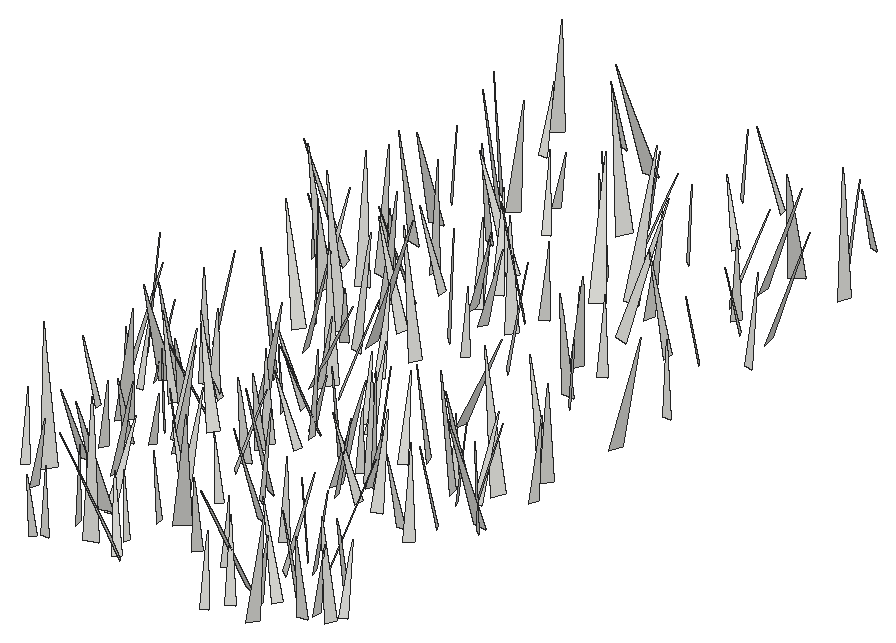
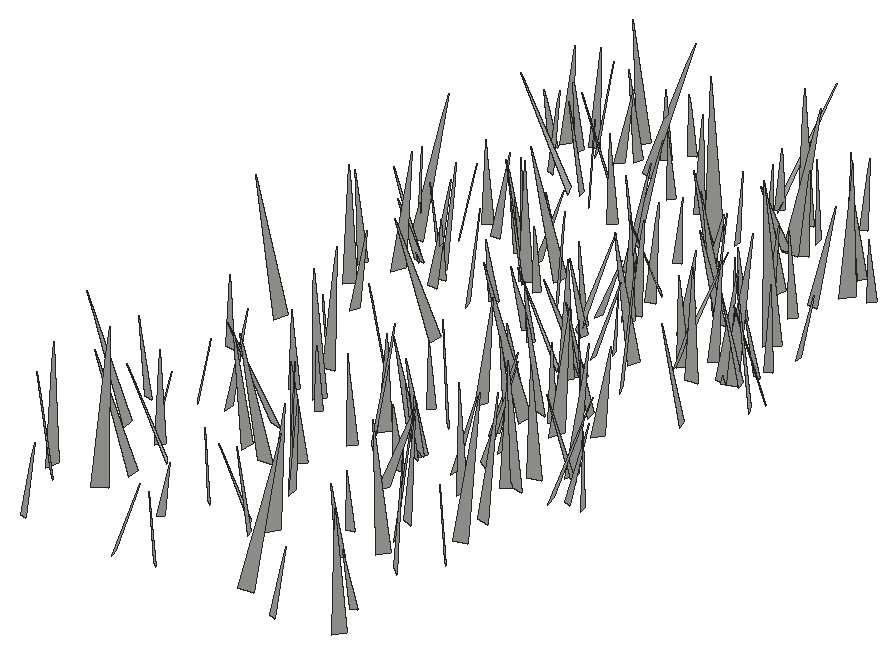
# SketchUp Ruby script. Lengths in inches.
U = 1.inch
M = Sketchup.active_model
def pt(a) = Geom::Point3d.new(a.map { |v| v * U })
def face(e, loops, mat)
  f = e.add_face(loops[0].map { |a| pt(a) })
  loops[1..].each { |l| e.add_face(l.map { |a| pt(a) }).erase! }
  f.material = f.back_material = mat if mat
  f
end
# faces: each face lists its corners as indices into pts; further lists are holes
def faces(e, pts, list, mat = nil) = list.each { |f| face(e, (f[0].is_a?(Array) ? f : [f]).map { |l| l.map { |i| pts[i] } }, mat) }
# xy, xz, yz: faces in a plane at the given z, y or x. An outline is a flat list of corners, or four numbers for a rectangle; further outlines are holes
def ring(l) = l.size == 4 ? [[l[0], l[1]], [l[2], l[1]], [l[2], l[3]], [l[0], l[3]]] : l.each_slice(2).to_a
def flat(e, list, mat, &to3) = list.each { |f| face(e, (f[0].is_a?(Array) ? f : [f]).map { |l| ring(l).map { |u, v| to3.(u, v) } }, mat) }
def xy(e, z, list, mat = nil) = flat(e, list, mat) { |x, y| [x, y, z] }
def xz(e, y, list, mat = nil) = flat(e, list, mat) { |x, z| [x, y, z] }
def yz(e, x, list, mat = nil) = flat(e, list, mat) { |y, z| [x, y, z] }
def lines(e, pts, list) = list.each { |a, b| e.add_line(pt(pts[a]), pt(pts[b])) }
# prism: a flat outline (further loops are holes) pulled along v
def prism(e, loops, v, mat = nil)
  f = face(e, loops, mat); d = Geom::Vector3d.new(v.map { |x| x * U })
  f.pushpull(f.normal.samedirection?(d) ? d.length : -d.length)
end
def box(e, o, s, mat = nil) = prism(e, [[o, [o[0] + s[0], o[1], o[2]], [o[0] + s[0], o[1] + s[1], o[2]], [o[0], o[1] + s[1], o[2]]]], [0, 0, s[2]], mat)
def at(x, y, z, deg = 0) = Geom::Transformation.translation(pt([x, y, z])) * Geom::Transformation.rotation(ORIGIN, Z_AXIS, deg.degrees)
def axes(o, x, y, z) = Geom::Transformation.new([*x, 0, *y, 0, *z, 0, *pt(o).to_a, 1])
def part(name) = M.definitions.add(name)
# library, detail: a bought-in or finely detailed component or shape, given as its bounding box
def library(name, o, s) = part(name).tap { |d| box(d.entities, o, s) }
def detail(e, o, s) = box(e.add_group.entities, o, s)
def put(e, d, t, mat = nil) = e.add_instance(d, t).tap { |i| i.material = mat if mat }
def group(e, t, mat = nil) = e.add_group.tap { |g| g.transformation = t; g.material = mat if mat }.entities
root = M.entities
c1 = part("fur_instance\#9")
p = [[0.8125,0,1.79],[0.67,-0.02,1.48],[0,-0.11,0],[0,0.11,0]]
faces(c1.entities,p,[[0,1,2,3]])
put(root,c1,axes([502.12,222.47,-21.66],[3.8396,0.83392,1.68617],[0.96833,-4.16197,-0.14664],[-1.61273,-0.51356,3.92638]))
put(root,c1,axes([501.79,197.2,-21.66],[5.69134,3.55142,2.30083],[3.82093,-5.97012,-0.23634],[-1.81848,-1.42926,6.70433]))
put(root,c1,axes([501.6,195.12,-21.66],[3.62165,4.35293,0.90177],[4.41878,-3.65214,-0.11732],[-0.48531,-0.76904,5.66132]))
put(root,c1,axes([505.58,223.1,-21.66],[-6.60705,-1.5953,0.55499],[-1.61141,6.62494,-0.14037],[0.50631,0.26714,6.79547]))
put(root,c1,axes([504,222.55,-21.66],[-1.28236,-4.10189,0.60594],[-4.14572,1.27987,-0.10961],[0.07509,0.61118,4.29626]))
put(root,c1,axes([504.39,186.52,-21.66],[-3.7389,-0.44853,0.79303],[-0.43438,3.82202,0.11371],[0.80087,-0.02096,3.764]))
put(root,c1,axes([505.36,191.68,-21.66],[0.0321,3.78164,0.61426],[3.82721,-0.05969,0.16749],[-0.17489,-0.6122,3.77806]))
put(root,c1,axes([505.9,173.29,-21.66],[-2.49672,2.92464,0.96124],[2.97957,2.60694,-0.1927],[0.77439,-0.6012,3.84057]))
put(root,c1,axes([505.07,190.25,-21.66],[1.42662,-4.11071,0.89066],[-4.20545,-1.41051,0.22612],[-0.07357,0.91596,4.34535]))
put(root,c1,axes([505.23,256.11,-21.66],[-4.12278,4.06528,3.37823],[4.64279,4.83304,-0.14992],[2.52655,-2.24755,5.78803]))
put(root,c1,axes([507.04,218.04,-21.66],[-7.37907,1.498,2.27835],[1.63074,7.6926,0.22378],[2.18531,-0.6822,7.52626]))
put(root,c1,axes([505.83,239.01,-21.66],[3.13173,2.6382,1.54856],[2.8558,-3.31576,-0.12654],[-1.0966,-1.10068,4.0929]))
put(root,c1,axes([505.16,203.51,-21.66],[5.01565,1.80166,1.23073],[1.89818,-5.12441,-0.23415],[-1.07592,-0.64182,5.32428]))
put(root,c1,axes([505.49,193.93,-21.66],[4.51759,1.55237,1.02195],[1.60919,-4.61101,-0.10928],[-0.92991,-0.4377,4.77562]))
put(root,c1,axes([507.41,194.6875,-21.66],[-0.73911,-5.79285,1.55471],[-5.99778,0.70592,-0.22109],[-0.03032,1.57006,5.83563]))
put(root,c1,axes([506.45,218.625,-21.66],[2.03381,4.83721,0.83738],[4.90479,-2.04045,-0.1258],[-0.20703,-0.82108,5.24587]))
put(root,c1,axes([507.09,251.49,-21.66],[-0.85461,3.70026,0.75554],[3.7566,0.91253,-0.21994],[0.38824,-0.68446,3.79129]))
put(root,c1,axes([506.39,194.58,-21.66],[2.6634,-7.09113,0.13913],[-7.08626,-2.66678,-0.26525],[-0.29724,0.03689,7.57017]))
put(root,c1,axes([508.29,174.0625,-21.66],[5.58768,-4.04107,3.86555],[-4.58295,-6.44048,-0.10822],[-3.20457,2.16447,6.89498]))
put(root,c1,axes([508.18,230.33,-21.66],[-1.31696,-6.51866,1.83434],[-6.75362,1.40125,0.13086],[0.49623,1.77078,6.64907]))
put(root,c1,axes([509.93,210.38,-21.66],[-5.57386,3.34507,0.61319],[3.34749,5.6042,-0.14346],[0.5998,-0.19191,6.49898]))
put(root,c1,axes([508.77,243.03,-21.66],[-4.32305,-4.69404,2.5219],[-5.10648,4.57733,-0.23372],[1.52244,2.02405,6.37716]))
put(root,c1,axes([507.38,234.79,-21.66],[2.10072,-7.09935,0.00934],[-7.09522,-2.09917,0.25546],[0.24231,0.08144,7.39923]))
put(root,c1,axes([509.6,191.54,-21.66],[-4.39525,1.44739,0.73649],[1.42922,4.45652,-0.22883],[0.77116,-0.01,4.62177]))
put(root,c1,axes([509.51,220.71,-21.66],[-2.53684,6.34204,1.9532],[6.60869,2.60398,0.12835],[0.60133,-1.86275,6.82939]))
put(root,c1,axes([509.66,196.33,-21.66],[-1.05184,5.80364,2.59591],[6.34975,1.09094,0.13387],[0.3189,-2.57972,5.89666]))
put(root,c1,axes([509.59,223.4375,-21.66],[-1.17344,-6.36654,3.3674],[-7.15717,1.41187,0.17527],[0.80444,3.27459,6.4714]))
put(root,c1,axes([509.77,177.61,-21.66],[-0.22883,-5.12281,0.23524],[-5.12454,0.23734,0.18366],[0.19416,0.22665,5.12463]))
put(root,c1,axes([507.93,186.05,-21.66],[6.18232,-5.30847,0.7026],[-5.32058,-6.21081,-0.10875],[-0.60412,0.37485,8.14795]))
put(root,c1,axes([510.06,212.77,-21.66],[4.77754,4.17311,2.72058],[4.61145,-5.13068,-0.22808],[-1.8844,-1.97551,6.33938]))
put(root,c1,axes([509.375,170.44,-21.66],[4.26328,-1.39926,0.74192],[-1.39292,-4.32659,-0.15583],[-0.75375,0.08115,4.48433]))
put(root,c1,axes([509.79,180.55,-21.66],[3.72524,-2.31212,0.81738],[-2.32656,-3.80205,-0.15146],[-0.77532,0.29988,4.38182]))
put(root,c1,axes([510.38,192.11,-21.66],[2.722,-4.21365,0.18087],[-4.20663,-2.72794,-0.24377],[-0.30292,0.01939,5.01046]))
put(root,c1,axes([512.64,195.01,-21.66],[-3.89073,-0.42692,0.42553],[-0.44504,3.90915,-0.14719],[0.40654,0.19356,3.91132]))
put(root,c1,axes([510.63,223.72,-21.66],[2.81621,-4.35059,0.38195],[-4.36621,-2.81499,0.12899],[-0.09891,0.39082,5.18093]))
put(root,c1,axes([513.21,212.65,-21.66],[-7.4138,3.10521,1.79195],[3.13289,7.61249,-0.22981],[1.74312,-0.47482,8.03455]))
put(root,c1,axes([511.11,182.79,-21.66],[1.53045,-4.60076,0.23907],[-4.60681,-1.52625,0.11946],[0.03806,0.26453,4.84716]))
put(root,c1,axes([512.83,238.01,-21.66],[-6.35073,-3.49942,2.22612],[-3.7296,6.59945,-0.26567],[1.81428,1.31702,7.24617]))
put(root,c1,axes([512.32,257.58,-21.66],[-1.30736,-3.53096,1.01989],[-3.67333,1.2908,-0.2398],[0.12042,1.04076,3.75757]))
put(root,c1,axes([512.32,186.76,-21.66],[2.78644,2.89477,1.9564],[3.12581,-3.18339,0.25829],[-1.56092,-1.20736,4.00964]))
put(root,c1,axes([512.07,194.68,-21.66],[-2.98009,3.50221,2.17702],[3.82104,3.35523,-0.16707],[1.55067,-1.53712,4.59549]))
put(root,c1,axes([511.69,241.23,-21.66],[5.17414,-4.36417,1.70527],[-4.54977,-5.28673,0.27499],[-1.1196,1.31532,6.76329]))
put(root,c1,axes([513.2,227.26,-21.66],[5.69837,-0.41307,2.53776],[-0.52377,-6.22748,0.16244],[-2.51724,0.36068,5.71101]))
put(root,c1,axes([513.98,201.78,-21.66],[-6.04607,-3.24149,2.31572],[-3.3744,6.40425,0.15438],[2.11738,0.95032,6.85845]))
put(root,c1,axes([514.81,190.72,-21.66],[-3.4454,-3.89131,0.03074],[-3.88746,3.44363,0.20759],[0.17579,-0.11462,5.19326]))
put(root,c1,axes([513.71,235.02,-21.66],[-1.84582,-5.09705,1.94608],[-5.40108,1.99766,0.10933],[0.77171,1.78987,5.41987]))
put(root,c1,axes([515.09,221.63,-21.66],[-2.82637,-5.01502,0.69558],[-5.06125,2.81969,-0.23605],[0.13409,0.7222,5.75179]))
put(root,c1,axes([513.14,184,-21.66],[3.09975,-1.98369,0.33098],[-1.98147,-3.11644,-0.1208],[-0.34401,0.07615,3.67817]))
put(root,c1,axes([513.58,219.08,-21.66],[6.28963,-0.96384,2.1084],[-1.07131,-6.61487,0.17192],[-2.05588,0.49827,6.36073]))
put(root,c1,axes([513.03,207.68,-21.66],[5.83146,1.27805,1.15338],[1.33487,-5.92923,-0.17895],[-1.08712,-0.42484,5.96719]))
put(root,c1,axes([516.1,189.5625,-21.66],[-4.785,3.6619,0.62252],[3.69492,4.79647,0.18627],[0.38032,-0.52686,6.02254]))
put(root,c1,axes([515.35,218.59,-21.66],[-3.60239,-0.15597,0.87969],[-0.19043,3.7046,-0.12301],[0.87288,0.16452,3.60367]))
put(root,c1,axes([514.49,185.8,-21.66],[0.1573,5.82785,1.1486],[5.93788,-0.12389,-0.18455],[0.15705,-1.15268,5.82705]))
put(root,c1,axes([513.8,177.32,-21.66],[5.74343,-0.59024,1.12729],[-0.57342,-5.85294,-0.14303],[-1.13593,-0.02976,5.77191]))
put(root,c1,axes([516.35,224.46,-21.66],[-4.66446,-0.17714,0.77084],[-0.14932,4.72517,0.1823],[0.77671,-0.15541,4.66426]))
put(root,c1,axes([515.3,162.77,-21.66],[2.03457,-2.99845,1.01926],[-3.06758,-2.16697,-0.25148],[-0.78708,0.69471,3.61482]))
put(root,c1,axes([514.53,244.33,-21.66],[2.97768,-2.23657,0.59018],[-2.29034,-2.98547,0.24174],[-0.32391,0.5494,3.71623]))
put(root,c1,axes([515.02,211.01,-21.66],[2.03296,-3.43324,0.36978],[-3.45285,-2.01606,0.26469],[0.04074,0.45292,3.9812]))
put(root,c1,axes([518.05,216.22,-21.66],[-5.4054,2.23783,0.44972],[2.26041,5.40869,0.2551],[0.31726,-0.40826,5.84475]))
put(root,c1,axes([517,239.64,-21.66],[-1.66344,3.87519,0.54462],[3.91265,1.65754,0.1564],[0.06977,-0.56232,4.21422]))
put(root,c1,axes([516.32,163.3125,-21.66],[0.16475,-3.83195,1.51207],[-4.1166,-0.0965,0.20397],[0.15418,1.51796,3.83006]))
put(root,c1,axes([516.62,170.34,-21.66],[2.27684,-3.73592,1.683],[-3.94498,-2.51908,-0.25488],[-1.10756,1.29258,4.36763]))
put(root,c1,axes([517.0625,210.37,-21.66],[1.06492,5.99669,1.55027],[6.17359,-1.15473,0.22589],[-0.50038,-1.48458,6.08632]))
put(root,c1,axes([515.94,184.25,-21.66],[6.14943,-1.42717,1.61929],[-1.52874,-6.3314,0.22535],[-1.52376,0.59247,6.30885]))
put(root,c1,axes([519.68,231.28,-21.66],[-6.207,1.9177,0.03314],[1.91765,6.20287,0.22937],[-0.03607,-0.22893,6.49244]))
put(root,c1,axes([517.23,167.34,-21.66],[4.14484,0.5886,1.74948],[0.68446,-4.48393,-0.11303],[-1.71425,-0.36717,4.1849]))
put(root,c1,axes([517.55,255.09,-21.66],[0.59961,-8.00132,0.48644],[-8.01433,-0.60861,-0.13198],[-0.1682,0.47514,8.02267]))
put(root,c1,axes([517.87,170.88,-21.66],[0.49777,-7.47829,0.86543],[-7.52286,-0.52678,-0.22508],[-0.28353,0.84808,7.49146]))
put(root,c1,axes([518.17,181.88,-21.66],[-3.06281,-3.15709,1.43812],[-3.29391,3.24851,0.11628],[1.08883,0.94666,4.3971]))
put(root,c1,axes([516.22,197.03,-21.66],[6.40795,-1.734,1.03011],[-1.73088,-6.48917,-0.15614],[-1.03535,0.11648,6.63658]))
put(root,c1,axes([518.39,170.79,-21.66],[-0.5351,4.97369,0.08314],[4.96853,0.53845,-0.2337],[0.24128,-0.05757,4.99693]))
put(root,c1,axes([519.27,203.65,-21.66],[-5.69,4.35692,2.08043],[4.49689,5.95288,-0.16772],[1.75752,-1.1258,7.16454]))
put(root,c1,axes([518.83,196.7,-21.66],[3.01328,1.01562,1.71575],[1.06477,-3.44849,0.1713],[-1.68569,-0.36275,3.17522]))
put(root,c1,axes([520.02,198.56,-21.66],[-4.58656,-0.99691,0.53395],[-0.9871,4.61746,0.14195],[0.55187,-0.02624,4.69151]))
put(root,c1,axes([518.82,202.57,-21.66],[4.01363,-0.60213,1.19124],[-0.70216,-4.16285,0.26162],[-1.13516,0.446,4.0501]))
put(root,c1,axes([520.74,227.54,-21.66],[-2.1836,4.82414,0.14178],[4.82373,2.17653,0.23433],[-0.15514,-0.2257,5.29014]))
put(root,c1,axes([517.41,212.3125,-21.66],[8.28106,0.30024,0.90595],[0.31898,-8.32832,-0.15571],[-0.89952,-0.18935,8.28504]))
put(root,c1,axes([520.34,165.41,-21.66],[1.64686,-6.77743,3.62945],[-7.62252,-1.92308,-0.13234],[-1.0018,3.49096,6.97339]))
put(root,c1,axes([518.03,202.4,-21.66],[5.44846,0.74036,0.07595],[0.73692,-5.44519,0.21553],[-0.10422,0.20337,5.4943]))
put(root,c1,axes([521.05,224.13,-21.66],[-1.86481,4.13252,0.34952],[4.14724,1.85655,0.17621],[-0.01744,-0.39104,4.53037]))
put(root,c1,axes([522.26,177.63,-21.66],[-3.36159,2.04077,0.19725],[2.04893,3.35754,0.1809],[0.07444,-0.25709,3.9284]))
put(root,c1,axes([520.93,224.73,-21.66],[1.65832,3.59632,1.35209],[3.82471,-1.68517,-0.20869],[-0.36513,-1.31848,3.95475]))
put(root,c1,axes([522.66,212.45,-21.66],[-6.31107,2.62453,1.38258],[2.63294,6.45317,-0.23139],[1.36651,-0.31261,6.83112]))
put(root,c1,axes([522,207.77,-21.66],[-1.31854,4.49628,0.43937],[4.51767,1.31381,0.11263],[0.01505,-0.45333,4.68427]))
put(root,c1,axes([522.85,244.4,-21.66],[-6.40886,3.74132,2.19702],[3.96061,6.64492,0.23769],[1.77143,-1.32114,7.41717]))
put(root,c1,axes([521.89,190.8125,-21.66],[4.08918,-3.36848,1.98263],[-3.52303,-4.41912,-0.24183],[-1.69286,1.05996,5.29241]))
put(root,c1,axes([520.69,223.88,-21.66],[4.88822,-0.89007,0.63341],[-0.87396,-4.92864,-0.18113],[-0.65546,-0.06625,4.96529]))
put(root,c1,axes([524.41,164.69,-21.66],[-5.605,-5.08718,0.25266],[-5.09303,5.60246,-0.18084],[0.06544,0.30374,7.56721]))
put(root,c1,axes([521.9,189.58,-21.66],[2.34766,-4.1804,1.05082],[-4.25289,-2.44131,-0.21062],[-0.70205,0.80976,4.78987]))
put(root,c1,axes([522.34,177.19,-21.66],[-0.07417,5.83715,1.21265],[5.95855,0.11247,-0.17697],[0.19614,-1.2097,5.83493]))
put(root,c1,axes([523.06,167.54,-21.66],[3.01506,-0.72225,2.0256],[-1.00024,-3.559,0.21985],[-1.90373,0.72607,3.09256]))
put(root,c1,axes([522.46,186.6875,-21.66],[1.7038,-4.78318,1.39426],[-4.94528,-1.80274,-0.14134],[-0.60574,1.26373,5.0756]))
put(root,c1,axes([522.62,217.67,-21.66],[3.82157,4.19761,2.25189],[4.45533,-4.17126,0.21447],[-1.68552,-1.50865,5.67259]))
put(root,c1,axes([523.06,172.51,-21.66],[3.59976,0.06174,1.80471],[0.19659,-4.01441,-0.2548],[-1.79504,-0.31584,3.59126]))
put(root,c1,axes([521.3,202.43,-21.66],[4.74716,3.3592,0.52437],[3.38285,-4.75689,-0.1518],[-0.33985,-0.42721,5.81349]))
put(root,c1,axes([524.63,191.89,-21.66],[-3.98782,0.86871,0.11292],[0.87287,3.98492,0.16912],[0.07423,-0.18933,4.07783]))
put(root,c1,axes([524.17,195.71,-21.66],[-3.22391,-4.50813,0.36238],[-4.51102,3.23719,0.13952],[0.32445,0.21334,5.54053]))
put(root,c1,axes([524.11,164.65,-21.66],[-2.51117,3.39602,0.58609],[3.43959,2.51478,0.1658],[0.21361,-0.57041,4.22035]))
put(root,c1,axes([522.62,184.79,-21.66],[3.07177,3.42083,0.35758],[3.42072,-3.08846,0.16062],[-0.35863,-0.15826,4.59478]))
put(root,c1,axes([524.23,194.5625,-21.66],[4.53301,0.32886,1.81446],[0.26511,-4.88148,0.22244],[-1.82486,0.10775,4.53948]))
put(root,c1,axes([523.32,195.82,-21.66],[3.83276,-0.80553,0.30542],[-0.78769,-3.84079,-0.24507],[-0.34886,-0.17786,3.90882]))
put(root,c1,axes([524.24,246.2,-21.66],[4.12014,1.91723,1.34742],[2.03951,-4.27599,-0.15214],[-1.154,-0.71202,4.54182]))
put(root,c1,axes([525.3125,179.01,-21.66],[-2.21806,2.84038,1.31516],[3.07662,2.27502,0.2754],[0.57601,-1.21396,3.59328]))
put(root,c1,axes([523.41,221.9,-21.66],[4.86131,-2.02952,0.59697],[-2.06386,-4.87843,0.22145],[-0.46454,0.43544,5.26329]))
put(root,c1,axes([525.74,225.36,-21.66],[4.20893,3.73459,3.7879],[4.59902,-4.98198,-0.19834],[-2.67289,-2.69131,5.62342]))
put(root,c1,axes([526.03,237.31,-21.66],[-5.05567,-0.39861,1.84756],[-0.46846,5.37567,-0.1221],[1.83109,0.27472,5.06989]))
put(root,c1,axes([526.51,222.44,-21.66],[-4.60516,3.74944,1.60687],[3.84875,4.79672,-0.16237],[1.35183,-0.88372,5.93628]))
put(root,c1,axes([525.85,216.1,-21.66],[-2.23187,2.81976,1.51549],[3.01775,2.4697,-0.15093],[1.06816,-1.08561,3.59298]))
put(root,c1,axes([526.67,199.8,-21.66],[-1.83169,3.1238,0.57494],[3.14275,1.87858,-0.19441],[0.4602,-0.39568,3.61599]))
put(root,c1,axes([527.19,236.27,-21.66],[-5.46878,-3.64969,2.6695],[-4.02035,5.84198,-0.2491],[2.0696,1.70441,6.57007]))
put(root,c1,axes([525.56,244.35,-21.66],[3.83341,2.26597,0.28943],[2.28132,-3.82668,-0.25597],[-0.11822,-0.36786,4.44568]))
put(root,c1,axes([525.23,173.38,-21.66],[5.72891,-5.77899,0.7373],[-5.79412,-5.75966,-0.12335],[-0.60698,0.43635,8.13646]))
put(root,c1,axes([527.93,183.64,-21.66],[-2.71876,-5.31687,1.33657],[-5.469,2.73415,-0.24823],[0.3815,1.3048,5.9665]))
put(root,c1,axes([527.48,256.66,-21.66],[-2.04031,-2.94511,1.87891],[-3.25881,2.38849,0.20512],[1.25863,1.41005,3.57693]))
put(root,c1,axes([527.37,226.46,-21.66],[-2.45808,3.26284,2.53045],[3.74921,2.99751,-0.22312],[1.72995,-1.86016,4.07903]))
put(root,c1,axes([529.19,232.26,-21.66],[-4.20767,6.2047,0.57896],[6.20765,4.23458,-0.26697],[0.54635,-0.32858,7.49209]))
put(root,c1,axes([528.35,198.36,-21.66],[-1.52341,4.48001,0.30788],[4.47725,1.54034,-0.26007],[0.34571,-0.20714,4.72479]))
put(root,c1,axes([528.46,181.59,-21.66],[-2.24155,-3.80564,2.54295],[-4.42537,2.52493,-0.12217],[1.16862,2.26183,4.41503]))
put(root,c1,axes([529.07,192.81,-21.66],[4.09073,2.15745,2.5023],[2.51133,-4.61824,-0.12369],[-2.14694,-1.2913,4.62314]))
put(root,c1,axes([530.66,178.79,-21.66],[-1.81224,-5.34948,0.90018],[-5.42401,1.80193,-0.21131],[0.08596,0.92064,5.64415]))
put(root,c1,axes([529.62,170.23,-21.66],[3.06125,-3.87557,0.82155],[-3.90702,-3.12527,-0.1848],[-0.65588,0.52812,4.93529]))
put(root,c1,axes([532.06,257.3,-21.66],[-4.50006,-1.01814,0.39176],[-1.03948,4.50642,-0.22865],[0.331,0.31016,4.60813]))
put(root,c1,axes([531.14,243.83,-21.66],[2.46567,3.17158,1.58955],[3.37143,-2.69731,0.15219],[-1.10413,-1.15357,4.01439]))
put(root,c1,axes([530.82,216.44,-21.66],[-3.67972,-3.6806,3.42599],[-4.33109,4.47676,0.15761],[2.55458,2.28831,5.20214]))
put(root,c1,axes([531.77,234.31,-21.66],[-0.24232,8.0833,1.63068],[8.24361,0.27788,-0.15248],[0.20433,-1.625,8.08549]))
put(root,c1,axes([533.08,248.8,-21.66],[-2.90723,2.3787,0.42473],[2.40963,2.90345,0.23285],[0.1797,-0.4498,3.74913]))
put(root,c1,axes([532.21,191.95,-21.66],[-2.65217,1.9255,1.58872],[2.09556,2.97695,-0.10973],[1.35655,-0.83418,3.2756]))
put(root,c1,axes([533.58,169.59,-21.66],[-2.47,2.58512,1.49197],[2.74392,2.72878,-0.18549],[1.17462,-0.93843,3.57063]))
put(root,c1,axes([534.37,195.92,-21.66],[-2.34195,3.99616,0.3444],[3.99913,2.35703,-0.15486],[0.30802,-0.21845,4.62925]))
put(root,c1,axes([533.28,187.12,-21.66],[4.00682,1.30969,1.18737],[1.29487,-4.17692,0.23764],[-1.20352,-0.13365,4.20874]))
put(root,c1,axes([531.96,188.66,-21.66],[6.74375,-1.56753,0.95704],[-1.61805,-6.79399,0.27364],[-0.86892,0.48558,6.91813]))
put(root,c1,axes([534.09,223.15,-21.66],[2.31719,-2.3997,1.71249],[-2.74416,-2.55172,0.13746],[-1.07739,1.33819,3.33302]))
put(root,c1,axes([535.8,187.33,-21.66],[-4.77809,0.40303,0.49366],[0.4272,4.79644,0.21897],[0.47289,-0.2608,4.79006]))
put(root,c1,axes([534.39,190.95,-21.66],[-1.98157,5.41612,3.08152],[6.10168,2.34277,-0.19399],[1.26474,-2.81671,5.76397]))
put(root,c1,axes([534.94,176.91,-21.66],[-2.61332,3.50076,2.27341],[3.90248,3.00092,-0.13507],[1.48133,-1.72983,4.36652]))
put(root,c1,axes([535.08,190.47,-21.66],[-2.81459,-5.30869,2.75415],[-5.79641,3.17103,0.18862],[1.47279,2.33491,6.00571]))
put(root,c1,axes([534.64,191.17,-21.66],[5.13574,3.88277,2.0176],[4.11622,-5.34233,-0.19668],[-1.48436,-1.3806,6.4353]))
put(root,c1,axes([535.89,198,-21.66],[4.40996,1.53054,2.75088],[1.88618,-5.07543,-0.19988],[-2.52036,-1.1203,4.66373]))
put(root,c1,axes([535.05,233,-21.66],[5.91491,-0.67607,1.90084],[-0.77835,-6.19702,0.21795],[-1.8613,0.44302,5.94943]))
put(root,c1,axes([534.76,190.34,-21.66],[3.71508,-1.29272,0.27873],[-1.28155,-3.72443,-0.19222],[-0.32626,-0.0905,3.92887]))
put(root,c1,axes([535.55,227.99,-21.66],[2.14003,7.20036,0.0672],[7.19519,-2.14104,0.27303],[-0.28086,0.01341,7.50668]))
put(root,c1,axes([534.06,205.3,-21.66],[6.32443,-0.86949,0.03215],[-0.87008,-6.31952,0.24926],[0.00213,0.25131,6.37905]))
put(root,c1,axes([537.27,161.76,-21.66],[-1.47,3.64091,0.87512],[3.73843,1.4809,0.11844],[0.21496,-0.85654,3.92467]))
put(root,c1,axes([535.49,221.23,-21.66],[5.23742,-3.794,0.7561],[-3.79638,-5.28528,-0.22367],[-0.74406,0.26094,6.46336]))
put(root,c1,axes([538.22,167.47,-21.66],[-2.55623,-6.61752,0.06611],[-6.61278,2.55692,0.25211],[0.25899,-0.02922,7.08959]))
put(root,c1,axes([538.65,163.96,-21.66],[-2.21571,3.96483,0.99922],[4.07213,2.24229,0.13245],[0.36886,-0.93805,4.54001]))
put(root,c1,axes([538.38,186.94,-21.66],[-2.22109,4.73282,1.14399],[4.81333,2.32397,-0.26934],[0.73496,-0.91711,5.22114]))
put(root,c1,axes([538.64,221.27,-21.66],[-2.37433,3.47563,1.70417],[3.72029,2.6012,-0.12184],[1.06942,-1.33243,4.20745]))
put(root,c1,axes([538.45,216.23,-21.66],[0.4786,-6.17329,1.68247],[-6.39725,-0.42884,0.2463],[0.12453,1.69584,6.18692]))
put(root,c1,axes([539,175.5,-21.66],[-3.54566,-2.66431,1.6705],[-2.78653,3.82874,0.19209],[1.45754,0.83849,4.43096]))
put(root,c1,axes([538.85,172,-21.66],[-2.72966,-3.54913,3.67888],[-4.47058,3.67982,0.23296],[2.47878,2.72838,4.47136]))
put(root,c1,axes([539.9375,214.6,-21.66],[-2.43911,-2.15453,1.73505],[-2.51562,2.68975,-0.19638],[1.15067,1.31336,3.24849]))
put(root,c1,axes([541.13,228.21,-21.66],[-5.71627,0.02456,1.51927],[0.09668,5.9079,0.26822],[1.51639,-0.28405,5.71003]))
put(root,c1,axes([541.875,167.17,-21.66],[-4.34264,3.05124,0.46122],[3.07623,4.34339,0.23041],[0.24406,-0.45414,5.3024]))
put(root,c1,axes([540.88,195.7,-21.66],[-1.02276,3.4571,1.0392],[3.60758,1.01767,0.16502],[0.12981,-1.04418,3.60144]))
put(root,c1,axes([540.79,197.32,-21.66],[-1.08369,-5.40972,1.03151],[-5.49173,1.14023,0.21038],[0.41232,0.96864,5.51318]))
put(root,c1,axes([541.58,194.57,-21.66],[-6.14594,-1.15799,1.95321],[-1.28361,6.42082,-0.2323],[1.87305,0.60056,6.24977]))
put(root,c1,axes([539.4,239.95,-21.66],[4.3993,3.63087,0.47155],[3.65139,-4.40515,-0.14642],[-0.27004,-0.41338,5.70225]))
put(root,c1,axes([540.69,165.73,-21.66],[4.29298,-1.68508,0.76366],[-1.68331,-4.35833,-0.1541],[-0.76754,0.13347,4.60928]))
put(root,c1,axes([540.94,174.16,-21.66],[4.61454,1.12705,1.27743],[1.23829,-4.75228,-0.2803],[-1.16993,-0.58453,4.7419]))
put(root,c1,axes([542.07,186,-21.66],[0.17037,-4.40384,1.04145],[-4.5148,-0.2364,-0.26107],[-0.30825,1.02847,4.3994]))
put(root,c1,axes([541.86,237.86,-21.66],[3.93082,-2.70083,1.38603],[-2.7651,-4.12134,-0.18897],[-1.2529,0.6221,4.76552]))
put(root,c1,axes([540.26,243.99,-21.66],[6.68807,0.43229,0.66728],[0.41432,-6.71942,0.20043],[-0.67859,0.15798,6.69903]))
put(root,c1,axes([541.15,248.11,-21.66],[4.3126,-6.65441,0.44802],[-6.65528,-4.32849,-0.22777],[-0.435,0.25174,7.9264]))
put(root,c1,axes([543.77,205.48,-21.66],[-4.87029,1.64927,0.93909],[1.65484,4.95663,-0.12272],[0.92923,-0.18296,5.1405]))
put(root,c1,axes([543.72,236.14,-21.66],[-3.07283,-1.79032,0.75021],[-1.87261,3.10397,-0.26279],[0.51124,0.60869,3.54662]))
put(root,c1,axes([543.37,257.13,-21.66],[-0.97443,-3.66118,0.75209],[-3.71136,1.03977,0.25308],[0.44234,0.6588,3.78017]))
put(root,c1,axes([542.37,162.77,-21.66],[5.43979,-3.16023,1.66658],[-3.30816,-5.60189,0.17546],[-1.34931,0.9938,6.28869]))
put(root,c1,axes([543.2,193.14,-21.66],[3.76786,2.01641,1.4087],[2.07515,-3.9894,0.15999],[-1.32064,-0.51569,4.27049]))
put(root,c1,axes([544.28,229.0625,-21.66],[-2.57629,-2.49445,0.93197],[-2.62206,2.60252,-0.28257],[0.46438,0.85602,3.57488]))
put(root,c1,axes([544.71,167.24,-21.66],[-4.89111,-2.11302,1.38613],[-2.21595,5.03778,-0.13961],[1.21481,0.68196,5.3262]))
put(root,c1,axes([544.7,188.27,-21.66],[-3.48684,-2.54111,1.02639],[-2.66037,3.53733,-0.28017],[0.65812,0.83597,4.30544]))
put(root,c1,axes([544.28,184.41,-21.66],[-3.13208,3.88614,1.48189],[4.03166,3.29255,-0.11327],[1.02167,-1.07935,4.98991]))
put(root,c1,axes([545.4,196.83,-21.66],[-6.9298,2.98954,1.57704],[3.02348,7.09089,-0.15622],[1.51094,-0.47802,7.54553]))
put(root,c1,axes([542.21,174.46,-21.66],[6.025,3.41302,0.55167],[3.40656,-6.04972,0.22351],[-0.59027,-0.07668,6.92094]))
put(root,c1,axes([544.89,194.19,-21.66],[0.14678,4.73777,0.12743],[4.7339,-0.15274,0.22615],[-0.23006,-0.12022,4.73465]))
put(root,c1,axes([545.87,172.86,-21.66],[-1.67476,-3.89018,1.26522],[-4.03938,1.78862,0.15259],[0.64624,1.09838,4.23261]))
put(root,c1,axes([545.64,166.3,-21.66],[1.04102,-4.92803,1.21287],[-5.07408,-1.03535,0.14838],[-0.10125,1.21771,5.0346]))
put(root,c1,axes([544.89,194.09,-21.66],[4.65489,2.00226,0.76997],[2.06003,-4.68544,-0.26978],[-0.59848,-0.55448,5.06006]))
put(root,c1,axes([546.18,249.22,-21.66],[3.88828,4.27161,1.82836],[4.44707,-4.1121,0.14976],[-1.3465,-1.2459,5.77433]))
put(root,c1,axes([546.34,167.6875,-21.66],[4.13906,-0.88394,1.08396],[-0.87234,-4.27812,-0.15771],[-1.09332,0.06702,4.22946]))
put(root,c1,axes([547.39,247.61,-21.66],[6.19428,-1.57461,3.33029],[-1.87234,-6.95675,0.19327],[-3.17247,1.03131,6.38836]))
put(root,c1,axes([548.3,167.4,-21.66],[-4.8782,2.33838,1.88669],[2.5546,5.12175,0.25721],[1.58166,-1.06025,5.40358]))
put(root,c1,axes([547.74,191.03,-21.66],[-0.40558,-7.48594,0.6627],[-7.51279,0.42075,0.15485],[0.19107,0.65318,7.49532]))
put(root,c1,axes([547.42,201.74,-21.66],[-3.8078,3.44308,3.43375],[4.19662,4.52997,0.11149],[2.45637,-2.40193,5.13242]))
put(root,c1,axes([548.35,189.96,-21.66],[-3.07714,-3.38347,1.94932],[-3.73457,3.27489,-0.21099],[1.14047,1.59489,4.5686]))
put(root,c1,axes([548.5,218.86,-21.66],[-0.06677,3.94377,1.582],[4.24655,0.00562,0.16522],[-0.15123,-1.5834,3.94087]))
put(root,c1,axes([548.48,231.44,-21.66],[0.70725,4.81258,1.31899],[4.97344,-0.78845,0.21001],[-0.40688,-1.27212,4.85974]))
put(root,c1,axes([548.76,168.73,-21.66],[-1.59242,3.59476,0.56652],[3.61736,1.63113,-0.18207],[0.39739,-0.44291,3.92746]))
put(root,c1,axes([546.8,236.7,-21.66],[7.02887,1.41814,0.69885],[1.44367,-7.05544,-0.2028],[-0.64447,-0.3379,7.16763]))
put(root,c1,axes([548.86,197.93,-21.66],[4.44334,-1.86269,1.64457],[-2.02269,-4.66849,0.17731],[-1.44323,0.80817,4.81471]))
put(root,c1,axes([548.43,211.14,-21.66],[6.87118,-2.4682,1.14103],[-2.53265,-6.93781,0.24398],[-0.98977,0.61792,7.29696]))
